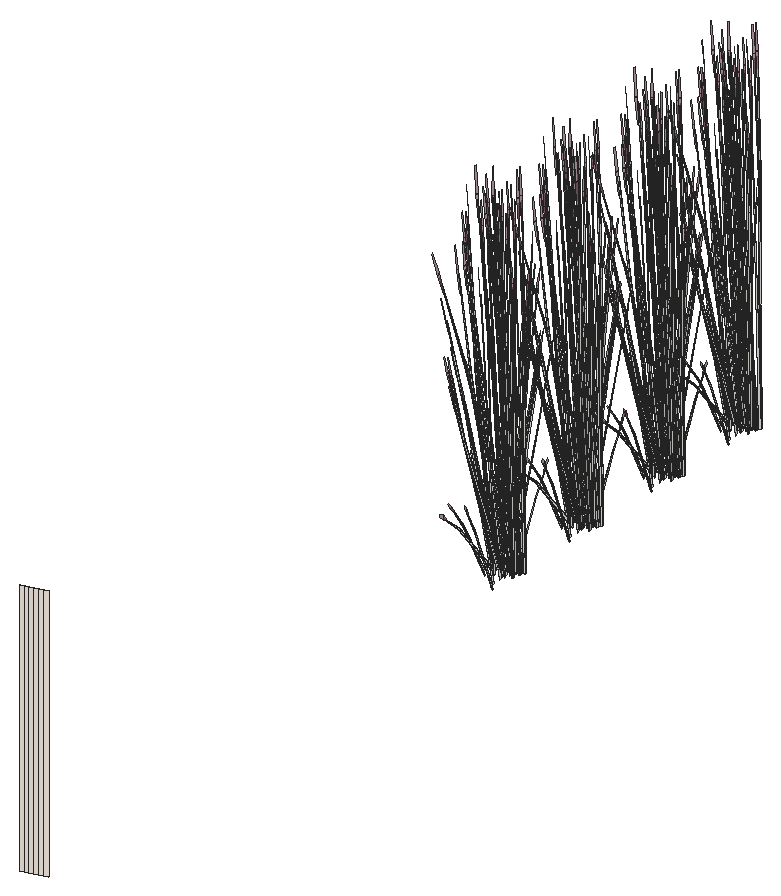
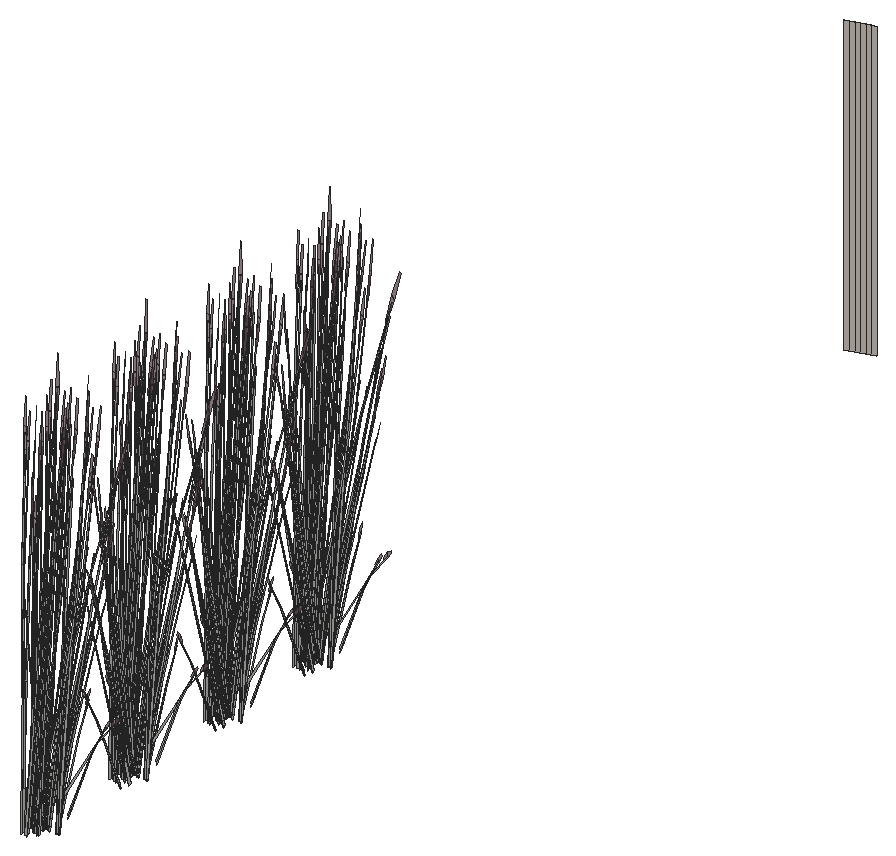
# SketchUp Ruby script. Lengths in inches.
U = 1.inch
M = Sketchup.active_model
def pt(a) = Geom::Point3d.new(a.map { |v| v * U })
def face(e, loops, mat)
  f = e.add_face(loops[0].map { |a| pt(a) })
  loops[1..].each { |l| e.add_face(l.map { |a| pt(a) }).erase! }
  f.material = f.back_material = mat if mat
  f
end
# faces: each face lists its corners as indices into pts; further lists are holes
def faces(e, pts, list, mat = nil) = list.each { |f| face(e, (f[0].is_a?(Array) ? f : [f]).map { |l| l.map { |i| pts[i] } }, mat) }
# xy, xz, yz: faces in a plane at the given z, y or x. An outline is a flat list of corners, or four numbers for a rectangle; further outlines are holes
def ring(l) = l.size == 4 ? [[l[0], l[1]], [l[2], l[1]], [l[2], l[3]], [l[0], l[3]]] : l.each_slice(2).to_a
def flat(e, list, mat, &to3) = list.each { |f| face(e, (f[0].is_a?(Array) ? f : [f]).map { |l| ring(l).map { |u, v| to3.(u, v) } }, mat) }
def xy(e, z, list, mat = nil) = flat(e, list, mat) { |x, y| [x, y, z] }
def xz(e, y, list, mat = nil) = flat(e, list, mat) { |x, z| [x, y, z] }
def yz(e, x, list, mat = nil) = flat(e, list, mat) { |y, z| [x, y, z] }
def lines(e, pts, list) = list.each { |a, b| e.add_line(pt(pts[a]), pt(pts[b])) }
# prism: a flat outline (further loops are holes) pulled along v
def prism(e, loops, v, mat = nil)
  f = face(e, loops, mat); d = Geom::Vector3d.new(v.map { |x| x * U })
  f.pushpull(f.normal.samedirection?(d) ? d.length : -d.length)
end
def box(e, o, s, mat = nil) = prism(e, [[o, [o[0] + s[0], o[1], o[2]], [o[0] + s[0], o[1] + s[1], o[2]], [o[0], o[1] + s[1], o[2]]]], [0, 0, s[2]], mat)
def at(x, y, z, deg = 0) = Geom::Transformation.translation(pt([x, y, z])) * Geom::Transformation.rotation(ORIGIN, Z_AXIS, deg.degrees)
def axes(o, x, y, z) = Geom::Transformation.new([*x, 0, *y, 0, *z, 0, *pt(o).to_a, 1])
def part(name) = M.definitions.add(name)
# library, detail: a bought-in or finely detailed component or shape, given as its bounding box
def library(name, o, s) = part(name).tap { |d| box(d.entities, o, s) }
def detail(e, o, s) = box(e.add_group.entities, o, s)
def put(e, d, t, mat = nil) = e.add_instance(d, t).tap { |i| i.material = mat if mat }
def group(e, t, mat = nil) = e.add_group.tap { |g| g.transformation = t; g.material = mat if mat }.entities
root = M.entities
M.materials.add("C01_Vanilla_Cream").color = [255, 246, 235]
M.materials.add("LightPink_Translucent").color = [144, 107, 117]
M.materials["LightPink_Translucent"].alpha = 0.75
c1 = part("blade")
p = [[2.15,0.21,22],[0,0.17,0],[0.09,0.45,0],[2.18,0.31,22],[2.29,0.31,22],[0.38,0.45,0],
  [2.48,0.24,33],[2.49,0.24,33],[2.48,0.22,33]]
faces(c1.entities,p,[[0,1,2,3],[4,5,2,3],[6,3,4,7],[8,0,3,6]])
c2 = part("seeds")
p = [[0.3,-0.1,1.38],[-0.01,-0.03,1.59],[-0.01,-0.03,0.03],[0.14,-0.07,-0.07],[0.29,-0.03,3],[0.15,0.01,3.11]]
faces(c2.entities,p,[[0,1,2,3],[1,0,4,5]],"LightPink_Translucent")
c3 = part("blade with seeds")
put(c3.entities,c1,at(0,0,0))
put(c3.entities,c2,axes([2.4,0.25,30.99],[1.5799,-0.05474,1.17369],[-0.12525,1.92788,0.29478],[-0.07173,-0.02425,1.56792]))
p = [[339.93,12.43,654],[339.37,12.32,654],[339.37,12.32,690],[339.93,12.43,690],[340.48,12.57,654],[340.48,12.57,690],
  [341.02,12.71,654],[341.02,12.71,690],[341.5625,12.88,654],[341.5625,12.88,690],[342.1,13.0625,654],[342.1,13.0625,690],
  [342.625,13.26,654],[342.625,13.26,690]]
faces(root,p,[[0,1,2,3],[4,0,3,5],[6,4,5,7],[8,6,7,9],[10,8,9,11],[12,10,11,13]],"C01_Vanilla_Cream")
put(root,c3,axes([340.5625,124.2,657.71],[-0.33433,0.21811,-0.29039],[-0.31649,-0.24905,0.3749],[-0.04815,0.12654,0.71734]))
put(root,c3,axes([342.27,95.55,655.6875],[-0.33282,0.31137,-0.51129],[-0.41344,-0.28235,-0.13419],[-0.13336,0.07767,1.12859]))
put(root,c3,axes([342.27,109.15,655.6875],[-0.33282,0.31137,-0.51129],[-0.41344,-0.28235,-0.13419],[-0.13336,0.07767,1.12859]))
put(root,c3,axes([342.27,123.55,655.6875],[-0.33282,0.31137,-0.51129],[-0.41344,-0.28235,-0.13419],[-0.13336,0.07767,1.12859]))
put(root,c3,axes([342.27,137.04,655.6875],[-0.33282,0.31137,-0.51129],[-0.41344,-0.28235,-0.13419],[-0.13336,0.07767,1.12859]))
put(root,c3,axes([341.42,93.23,658.14],[0.07631,0.33368,0.29039],[-0.43626,0.08811,-0.3749],[-0.11718,-0.09562,0.71734]))
put(root,c3,axes([341.42,106.83,658.14],[0.07631,0.33368,0.29039],[-0.43626,0.08811,-0.3749],[-0.11718,-0.09562,0.71734]))
put(root,c3,axes([341.42,121.23,658.14],[0.07631,0.33368,0.29039],[-0.43626,0.08811,-0.3749],[-0.11718,-0.09562,0.71734]))
put(root,c3,axes([341.42,134.72,658.14],[0.07631,0.33368,0.29039],[-0.43626,0.08811,-0.3749],[-0.11718,-0.09562,0.71734]))
put(root,c3,axes([339.37,96.98,657.86],[0.05606,-0.02501,1.45454],[0.46332,0.16636,-0.13744],[-0.01089,0.13852,0.2574]))
put(root,c3,axes([339.37,110.58,657.86],[0.05606,-0.02501,1.45454],[0.46332,0.16636,-0.13744],[-0.01089,0.13852,0.2574]))
put(root,c3,axes([339.37,124.97,657.86],[0.05606,-0.02501,1.45454],[0.46332,0.16636,-0.13744],[-0.01089,0.13852,0.2574]))
put(root,c3,axes([340.42,94.53,655.91],[-0.45961,0.34828,0.2522],[-0.45989,-0.34462,-0.29923],[-0.01605,-0.09891,1.35206]))
put(root,c3,axes([340.42,108.13,655.91],[-0.45961,0.34828,0.2522],[-0.45989,-0.34462,-0.29923],[-0.01605,-0.09891,1.35206]))
put(root,c3,axes([340.42,122.52,655.91],[-0.45961,0.34828,0.2522],[-0.45989,-0.34462,-0.29923],[-0.01605,-0.09891,1.35206]))
put(root,c3,axes([340.42,136.01,655.91],[-0.45961,0.34828,0.2522],[-0.45989,-0.34462,-0.29923],[-0.01605,-0.09891,1.35206]))
put(root,c3,axes([342.3125,95.49,656.73],[0.427,0.16705,1.24034],[-0.41831,0.35988,0.49049],[-0.18737,-0.21329,1.03981]))
put(root,c3,axes([342.3125,109.09,656.73],[0.427,0.16705,1.24034],[-0.41831,0.35988,0.49049],[-0.18737,-0.21329,1.03981]))
put(root,c3,axes([342.3125,123.49,656.73],[0.427,0.16705,1.24034],[-0.41831,0.35988,0.49049],[-0.18737,-0.21329,1.03981]))
put(root,c3,axes([342.3125,136.98,656.73],[0.427,0.16705,1.24034],[-0.41831,0.35988,0.49049],[-0.18737,-0.21329,1.03981]))
put(root,c3,axes([340.68,92.46,656.27],[0.25775,0.14418,0.94186],[-0.37538,0.08667,0.69201],[-0.08032,-0.11081,0.20745]))
put(root,c3,axes([340.68,106.06,656.27],[0.25775,0.14418,0.94186],[-0.37538,0.08667,0.69201],[-0.08032,-0.11081,0.20745]))
put(root,c3,axes([340.68,120.46,656.27],[0.25775,0.14418,0.94186],[-0.37538,0.08667,0.69201],[-0.08032,-0.11081,0.20745]))
put(root,c3,axes([340.68,133.95,656.27],[0.25775,0.14418,0.94186],[-0.37538,0.08667,0.69201],[-0.08032,-0.11081,0.20745]))
put(root,c3,axes([342.5,95.375,656.02],[-0.48249,-0.33343,-0.20658],[0.406,-0.37441,0.45206],[-0.12993,0.039,1.37937]))
put(root,c3,axes([342.5,108.97,656.02],[-0.48249,-0.33343,-0.20658],[0.406,-0.37441,0.45206],[-0.12993,0.039,1.37937]))
put(root,c3,axes([342.5,123.37,656.02],[-0.48249,-0.33343,-0.20658],[0.406,-0.37441,0.45206],[-0.12993,0.039,1.37937]))
put(root,c3,axes([342.5,136.86,656.02],[-0.48249,-0.33343,-0.20658],[0.406,-0.37441,0.45206],[-0.12993,0.039,1.37937]))
put(root,c3,axes([341.625,95.06,655.8125],[-0.29683,-0.34771,-0.36686],[0.44961,-0.24485,0.17656],[-0.09606,-0.04302,1.17788]))
put(root,c3,axes([341.625,108.65,655.8125],[-0.29683,-0.34771,-0.36686],[0.44961,-0.24485,0.17656],[-0.09606,-0.04302,1.17788]))
put(root,c3,axes([341.625,123.05,655.8125],[-0.29683,-0.34771,-0.36686],[0.44961,-0.24485,0.17656],[-0.09606,-0.04302,1.17788]))
put(root,c3,axes([341.625,136.54,655.8125],[-0.29683,-0.34771,-0.36686],[0.44961,-0.24485,0.17656],[-0.09606,-0.04302,1.17788]))
put(root,c3,axes([340.78,95.97,658.38],[-0.01286,0.38319,-0.64665],[-0.54141,-0.02574,0.07804],[-0.05714,0.16234,0.91476]))
put(root,c3,axes([340.78,109.57,658.38],[-0.01286,0.38319,-0.64665],[-0.54141,-0.02574,0.07804],[-0.05714,0.16234,0.91476]))
put(root,c3,axes([340.78,123.97,658.38],[-0.01286,0.38319,-0.64665],[-0.54141,-0.02574,0.07804],[-0.05714,0.16234,0.91476]))
put(root,c3,axes([340.77,97.05,656.27],[-0.01279,-0.24632,0.94186],[0.31954,0.17569,0.69201],[-0.06284,0.11741,0.20745]))
put(root,c3,axes([340.77,110.65,656.27],[-0.01279,-0.24632,0.94186],[0.31954,0.17569,0.69201],[-0.06284,0.11741,0.20745]))
put(root,c3,axes([340.77,125.05,656.27],[-0.01279,-0.24632,0.94186],[0.31954,0.17569,0.69201],[-0.06284,0.11741,0.20745]))
put(root,c3,axes([341.22,92.84,658.18],[0.55043,-0.10648,0.44086],[0.09553,0.41768,0.3635],[-0.12945,-0.1231,0.91224]))
put(root,c3,axes([341.22,106.4375,658.18],[0.55043,-0.10648,0.44086],[0.09553,0.41768,0.3635],[-0.12945,-0.1231,0.91224]))
put(root,c3,axes([341.22,120.83,658.18],[0.55043,-0.10648,0.44086],[0.09553,0.41768,0.3635],[-0.12945,-0.1231,0.91224]))
put(root,c3,axes([341.22,134.33,658.18],[0.55043,-0.10648,0.44086],[0.09553,0.41768,0.3635],[-0.12945,-0.1231,0.91224]))
put(root,c3,axes([342.26,95.31,655.8125],[-0.53657,0.02557,-0.36686],[-0.04852,-0.4245,0.17656],[-0.09606,0.04302,1.17788]))
put(root,c3,axes([342.26,108.9,655.8125],[-0.53657,0.02557,-0.36686],[-0.04852,-0.4245,0.17656],[-0.09606,0.04302,1.17788]))
put(root,c3,axes([342.26,123.3,655.8125],[-0.53657,0.02557,-0.36686],[-0.04852,-0.4245,0.17656],[-0.09606,0.04302,1.17788]))
put(root,c3,axes([342.26,136.79,655.8125],[-0.53657,0.02557,-0.36686],[-0.04852,-0.4245,0.17656],[-0.09606,0.04302,1.17788]))
put(root,c3,axes([341.35,92.93,657.88],[0.22457,-0.26316,0.05273],[0.3198,0.15321,0.41509],[-0.10339,-0.08437,0.63295]))
put(root,c3,axes([341.35,106.53,657.88],[0.22457,-0.26316,0.05273],[0.3198,0.15321,0.41509],[-0.10339,-0.08437,0.63295]))
put(root,c3,axes([341.35,120.92,657.88],[0.22457,-0.26316,0.05273],[0.3198,0.15321,0.41509],[-0.10339,-0.08437,0.63295]))
put(root,c3,axes([341.35,134.42,657.88],[0.22457,-0.26316,0.05273],[0.3198,0.15321,0.41509],[-0.10339,-0.08437,0.63295]))
put(root,c3,axes([341.23,96.02,656.03],[0.46245,0.20713,0.40713],[-0.27641,0.37142,0],[-0.10533,-0.04718,1.29153]))
put(root,c3,axes([341.23,109.61,656.03],[0.46245,0.20713,0.40713],[-0.27641,0.37142,0],[-0.10533,-0.04718,1.29153]))
put(root,c3,axes([341.23,124.01,656.03],[0.46245,0.20713,0.40713],[-0.27641,0.37142,0],[-0.10533,-0.04718,1.29153]))
put(root,c3,axes([341.23,137.5,656.03],[0.46245,0.20713,0.40713],[-0.27641,0.37142,0],[-0.10533,-0.04718,1.29153]))
put(root,c3,axes([340.6,96.51,656.76],[0.01086,-0.21386,1.26563],[0.48828,0.11296,0.1749],[-0.04231,0.22792,0.59763]))
put(root,c3,axes([340.6,110.11,656.76],[0.01086,-0.21386,1.26563],[0.48828,0.11296,0.1749],[-0.04231,0.22792,0.59763]))
put(root,c3,axes([340.6,124.51,656.76],[0.01086,-0.21386,1.26563],[0.48828,0.11296,0.1749],[-0.04231,0.22792,0.59763]))
put(root,c3,axes([341.67,95.26,656],[0.13096,-0.49088,-0.19212],[0.62096,0.08557,0.42042],[-0.1085,-0.06779,1.28281]))
put(root,c3,axes([341.67,108.85,656],[0.13096,-0.49088,-0.19212],[0.62096,0.08557,0.42042],[-0.1085,-0.06779,1.28281]))
put(root,c3,axes([341.67,123.25,656],[0.13096,-0.49088,-0.19212],[0.62096,0.08557,0.42042],[-0.1085,-0.06779,1.28281]))
put(root,c3,axes([341.67,136.74,656],[0.13096,-0.49088,-0.19212],[0.62096,0.08557,0.42042],[-0.1085,-0.06779,1.28281]))
put(root,c3,axes([341.89,95.37,656.15],[-0.09532,0.36971,0.11873],[-0.46572,-0.06418,-0.33905],[-0.08476,-0.03796,1.0393]))
put(root,c3,axes([341.89,108.97,656.15],[-0.09532,0.36971,0.11873],[-0.46572,-0.06418,-0.33905],[-0.08476,-0.03796,1.0393]))
put(root,c3,axes([341.89,123.36,656.15],[-0.09532,0.36971,0.11873],[-0.46572,-0.06418,-0.33905],[-0.08476,-0.03796,1.0393]))
put(root,c3,axes([341.89,136.86,656.15],[-0.09532,0.36971,0.11873],[-0.46572,-0.06418,-0.33905],[-0.08476,-0.03796,1.0393]))
put(root,c3,axes([341.84,92.15,657.87],[-0.07558,-0.05808,1.43454],[-0.50436,0.03682,-0.22687],[-0.08049,-0.13892,0.11505]))
put(root,c3,axes([341.84,105.75,657.87],[-0.07558,-0.05808,1.43454],[-0.50436,0.03682,-0.22687],[-0.08049,-0.13892,0.11505]))
put(root,c3,axes([341.84,120.14,657.87],[-0.07558,-0.05808,1.43454],[-0.50436,0.03682,-0.22687],[-0.08049,-0.13892,0.11505]))
put(root,c3,axes([341.84,133.63,657.87],[-0.07558,-0.05808,1.43454],[-0.50436,0.03682,-0.22687],[-0.08049,-0.13892,0.11505]))
put(root,c3,axes([342.82,96.4,655.65],[-0.46245,0.20713,-0.40713],[-0.27641,-0.37142,0],[-0.10533,0.04718,1.29153]))
put(root,c3,axes([342.82,110,655.65],[-0.46245,0.20713,-0.40713],[-0.27641,-0.37142,0],[-0.10533,0.04718,1.29153]))
put(root,c3,axes([342.82,124.39,655.65],[-0.46245,0.20713,-0.40713],[-0.27641,-0.37142,0],[-0.10533,0.04718,1.29153]))
put(root,c3,axes([342.82,137.89,655.65],[-0.46245,0.20713,-0.40713],[-0.27641,-0.37142,0],[-0.10533,0.04718,1.29153]))
put(root,c3,axes([340.08,94.34,655.65],[0,-0.41426,-0.40713],[0.55282,0,0],[0,-0.09435,1.29153]))
put(root,c3,axes([340.08,107.94,655.65],[0,-0.41426,-0.40713],[0.55282,0,0],[0,-0.09435,1.29153]))
put(root,c3,axes([340.08,122.33,655.65],[0,-0.41426,-0.40713],[0.55282,0,0],[0,-0.09435,1.29153]))
put(root,c3,axes([340.08,135.82,655.65],[0,-0.41426,-0.40713],[0.55282,0,0],[0,-0.09435,1.29153]))
put(root,c3,axes([340.32,94.72,656.03],[0,0.41426,0.40713],[-0.55282,0,0],[0,-0.09435,1.29153]))
put(root,c3,axes([340.32,108.32,656.03],[0,0.41426,0.40713],[-0.55282,0,0],[0,-0.09435,1.29153]))
put(root,c3,axes([340.32,122.72,656.03],[0,0.41426,0.40713],[-0.55282,0,0],[0,-0.09435,1.29153]))
put(root,c3,axes([340.32,136.21,656.03],[0,0.41426,0.40713],[-0.55282,0,0],[0,-0.09435,1.29153]))
put(root,c3,axes([342.85,96.29,655.8],[-0.30508,-0.41657,-0.04217],[0.51685,-0.2315,0.42318],[-0.12736,0.03966,1.34177]))
put(root,c3,axes([342.85,109.89,655.8],[-0.30508,-0.41657,-0.04217],[0.51685,-0.2315,0.42318],[-0.12736,0.03966,1.34177]))
put(root,c3,axes([342.85,124.28,655.8],[-0.30508,-0.41657,-0.04217],[0.51685,-0.2315,0.42318],[-0.12736,0.03966,1.34177]))
put(root,c3,axes([342.85,137.77,655.8],[-0.30508,-0.41657,-0.04217],[0.51685,-0.2315,0.42318],[-0.12736,0.03966,1.34177]))
put(root,c3,axes([340.89,96.1,658.1],[0.35372,0.27835,-0.4651],[-0.37366,0.24377,-0.36026],[-0.05382,0.14142,0.88993]))
put(root,c3,axes([340.89,109.7,658.1],[0.35372,0.27835,-0.4651],[-0.37366,0.24377,-0.36026],[-0.05382,0.14142,0.88993]))
put(root,c3,axes([340.89,124.1,658.1],[0.35372,0.27835,-0.4651],[-0.37366,0.24377,-0.36026],[-0.05382,0.14142,0.88993]))
put(root,c3,axes([342.71,96.24,655.66],[-0.46099,-0.1025,-0.25402],[0.11607,-0.36097,0.25402],[-0.09293,0.04163,1.13959]))
put(root,c3,axes([342.71,109.84,655.66],[-0.46099,-0.1025,-0.25402],[0.11607,-0.36097,0.25402],[-0.09293,0.04163,1.13959]))
put(root,c3,axes([342.71,124.23,655.66],[-0.46099,-0.1025,-0.25402],[0.11607,-0.36097,0.25402],[-0.09293,0.04163,1.13959]))
put(root,c3,axes([342.71,137.72,655.66],[-0.46099,-0.1025,-0.25402],[0.11607,-0.36097,0.25402],[-0.09293,0.04163,1.13959]))
put(root,c3,axes([340.74,95.89,658.14],[0.33433,-0.21811,0.29039],[0.31649,0.24905,-0.3749],[-0.04815,0.12654,0.71734]))
put(root,c3,axes([340.74,109.49,658.14],[0.33433,-0.21811,0.29039],[0.31649,0.24905,-0.3749],[-0.04815,0.12654,0.71734]))
put(root,c3,axes([340.74,123.89,658.14],[0.33433,-0.21811,0.29039],[0.31649,0.24905,-0.3749],[-0.04815,0.12654,0.71734]))
put(root,c3,axes([340.74,137.38,658.14],[0.33433,-0.21811,0.29039],[0.31649,0.24905,-0.3749],[-0.04815,0.12654,0.71734]))
put(root,c3,axes([341.53,94.82,656.1875],[-0.55647,-0.19766,-0.23858],[0.26794,-0.4172,-0.41002],[-0.01749,-0.10243,1.3096]))
put(root,c3,axes([341.53,108.41,656.1875],[-0.55647,-0.19766,-0.23858],[0.26794,-0.4172,-0.41002],[-0.01749,-0.10243,1.3096]))
put(root,c3,axes([341.53,122.81,656.1875],[-0.55647,-0.19766,-0.23858],[0.26794,-0.4172,-0.41002],[-0.01749,-0.10243,1.3096]))
put(root,c3,axes([341.53,136.3,656.1875],[-0.55647,-0.19766,-0.23858],[0.26794,-0.4172,-0.41002],[-0.01749,-0.10243,1.3096]))
put(root,c3,axes([342.98,94.69,656.33],[-0.0135,-0.39004,1.15843],[0.61089,0.10111,0.49049],[-0.14449,0.21343,1.09347]))
put(root,c3,axes([342.98,108.29,656.33],[-0.0135,-0.39004,1.15843],[0.61089,0.10111,0.49049],[-0.14449,0.21343,1.09347]))
put(root,c3,axes([342.98,122.6875,656.33],[-0.0135,-0.39004,1.15843],[0.61089,0.10111,0.49049],[-0.14449,0.21343,1.09347]))
put(root,c3,axes([342.98,136.18,656.33],[-0.0135,-0.39004,1.15843],[0.61089,0.10111,0.49049],[-0.14449,0.21343,1.09347]))
put(root,c3,axes([340.52,95.95,658.43],[0.54305,0.02053,-0.11068],[-0.01484,0.38862,-0.61434],[-0.03772,0.14967,0.93347]))
put(root,c3,axes([340.52,109.55,658.43],[0.54305,0.02053,-0.11068],[-0.01484,0.38862,-0.61434],[-0.03772,0.14967,0.93347]))
put(root,c3,axes([340.52,123.95,658.43],[0.54305,0.02053,-0.11068],[-0.01484,0.38862,-0.61434],[-0.03772,0.14967,0.93347]))
put(root,c3,axes([340.51,96.52,656.31],[0.44888,-0.07336,0.05336],[0.1032,0.29555,-0.7077],[-0.02846,0.14961,0.63435]))
put(root,c3,axes([340.51,110.12,656.31],[0.44888,-0.07336,0.05336],[0.1032,0.29555,-0.7077],[-0.02846,0.14961,0.63435]))
put(root,c3,axes([340.51,124.51,656.31],[0.44888,-0.07336,0.05336],[0.1032,0.29555,-0.7077],[-0.02846,0.14961,0.63435]))
put(root,c3,axes([342.63,95.19,656.1875],[0.05758,0.4727,-0.23858],[-0.59969,0.02858,-0.41002],[-0.1056,0.06296,1.3096]))
put(root,c3,axes([342.63,108.79,656.1875],[0.05758,0.4727,-0.23858],[-0.59969,0.02858,-0.41002],[-0.1056,0.06296,1.3096]))
put(root,c3,axes([342.63,123.18,656.1875],[0.05758,0.4727,-0.23858],[-0.59969,0.02858,-0.41002],[-0.1056,0.06296,1.3096]))
put(root,c3,axes([342.63,136.67,656.1875],[0.05758,0.4727,-0.23858],[-0.59969,0.02858,-0.41002],[-0.1056,0.06296,1.3096]))
put(root,c3,axes([341.28,94.4,655.72],[-0.20292,-0.42481,-0.57265],[0.58453,-0.15299,-0.1503],[-0.02243,-0.14385,1.26402]))
put(root,c3,axes([341.28,107.99,655.72],[-0.20292,-0.42481,-0.57265],[0.58453,-0.15299,-0.1503],[-0.02243,-0.14385,1.26402]))
put(root,c3,axes([341.28,122.39,655.72],[-0.20292,-0.42481,-0.57265],[0.58453,-0.15299,-0.1503],[-0.02243,-0.14385,1.26402]))
put(root,c3,axes([341.28,135.88,655.72],[-0.20292,-0.42481,-0.57265],[0.58453,-0.15299,-0.1503],[-0.02243,-0.14385,1.26402]))
put(root,c3,axes([342.61,93.05,658.13],[-0.48353,0.19287,-0.09971],[-0.23761,-0.34232,-0.55346],[-0.0638,-0.14425,0.84097]))
put(root,c3,axes([342.61,106.64,658.13],[-0.48353,0.19287,-0.09971],[-0.23761,-0.34232,-0.55346],[-0.0638,-0.14425,0.84097]))
put(root,c3,axes([342.61,121.04,658.13],[-0.48353,0.19287,-0.09971],[-0.23761,-0.34232,-0.55346],[-0.0638,-0.14425,0.84097]))
put(root,c3,axes([342.61,134.53,658.13],[-0.48353,0.19287,-0.09971],[-0.23761,-0.34232,-0.55346],[-0.0638,-0.14425,0.84097]))
put(root,c3,axes([342.19,93.0625,657.84],[-0.48573,-0.10385,-0.41901],[0.16649,-0.35605,-0.32456],[-0.04454,-0.14335,0.80174]))
put(root,c3,axes([342.19,106.66,657.84],[-0.48573,-0.10385,-0.41901],[0.16649,-0.35605,-0.32456],[-0.04454,-0.14335,0.80174]))
put(root,c3,axes([342.19,121.06,657.84],[-0.48573,-0.10385,-0.41901],[0.16649,-0.35605,-0.32456],[-0.04454,-0.14335,0.80174]))
put(root,c3,axes([342.19,134.55,657.84],[-0.48573,-0.10385,-0.41901],[0.16649,-0.35605,-0.32456],[-0.04454,-0.14335,0.80174]))
put(root,c3,axes([341.3,95.7,657.18],[-0.01209,-0.159,1.40529],[0.52417,0.10548,0.11363],[-0.03242,0.22659,0.60075]))
put(root,c3,axes([341.3,109.3,657.18],[-0.01209,-0.159,1.40529],[0.52417,0.10548,0.11363],[-0.03242,0.22659,0.60075]))
put(root,c3,axes([341.3,123.7,657.18],[-0.01209,-0.159,1.40529],[0.52417,0.10548,0.11363],[-0.03242,0.22659,0.60075]))
put(root,c3,axes([340.32,94.35,655.66],[0.34492,-0.25847,-0.25402],[0.34492,0.25847,0.25402],[0,-0.08325,1.13959]))
put(root,c3,axes([340.32,107.94,655.66],[0.34492,-0.25847,-0.25402],[0.34492,0.25847,0.25402],[0,-0.08325,1.13959]))
put(root,c3,axes([340.32,122.34,655.66],[0.34492,-0.25847,-0.25402],[0.34492,0.25847,0.25402],[0,-0.08325,1.13959]))
put(root,c3,axes([340.32,135.83,655.66],[0.34492,-0.25847,-0.25402],[0.34492,0.25847,0.25402],[0,-0.08325,1.13959]))
put(root,c3,axes([341.875,92.67,655.74],[-0.34145,0.23766,-0.03192],[-0.31287,-0.26029,-0.14473],[-0.02203,-0.07375,0.47736]))
put(root,c3,axes([341.875,106.27,655.74],[-0.34145,0.23766,-0.03192],[-0.31287,-0.26029,-0.14473],[-0.02203,-0.07375,0.47736]))
put(root,c3,axes([341.875,120.67,655.74],[-0.34145,0.23766,-0.03192],[-0.31287,-0.26029,-0.14473],[-0.02203,-0.07375,0.47736]))
put(root,c3,axes([341.875,134.16,655.74],[-0.34145,0.23766,-0.03192],[-0.31287,-0.26029,-0.14473],[-0.02203,-0.07375,0.47736]))
put(root,c3,axes([341.74,95.02,655.9375],[0.62452,0.08728,0.37519],[-0.1271,0.49295,0.14723],[-0.09127,-0.0476,1.30262]))
put(root,c3,axes([341.74,108.62,655.9375],[0.62452,0.08728,0.37519],[-0.1271,0.49295,0.14723],[-0.09127,-0.0476,1.30262]))
put(root,c3,axes([341.74,123.01,655.9375],[0.62452,0.08728,0.37519],[-0.1271,0.49295,0.14723],[-0.09127,-0.0476,1.30262]))
put(root,c3,axes([341.74,136.5,655.9375],[0.62452,0.08728,0.37519],[-0.1271,0.49295,0.14723],[-0.09127,-0.0476,1.30262]))
put(root,c3,axes([341.58,94.93,656.23],[-0.23974,0.37328,0.36686],[-0.49814,-0.17965,-0.17656],[0,-0.08605,1.17788]))
put(root,c3,axes([341.58,108.53,656.23],[-0.23974,0.37328,0.36686],[-0.49814,-0.17965,-0.17656],[0,-0.08605,1.17788]))
put(root,c3,axes([341.58,122.92,656.23],[-0.23974,0.37328,0.36686],[-0.49814,-0.17965,-0.17656],[0,-0.08605,1.17788]))
put(root,c3,axes([341.58,136.41,656.23],[-0.23974,0.37328,0.36686],[-0.49814,-0.17965,-0.17656],[0,-0.08605,1.17788]))
put(root,c3,axes([342.37,93.13,658.08],[-0.23583,-0.33684,-0.58257],[0.48546,-0.18772,0.0703],[-0.05515,-0.16275,0.8241]))
put(root,c3,axes([342.37,106.73,658.08],[-0.23583,-0.33684,-0.58257],[0.48546,-0.18772,0.0703],[-0.05515,-0.16275,0.8241]))
put(root,c3,axes([342.37,121.125,658.08],[-0.23583,-0.33684,-0.58257],[0.48546,-0.18772,0.0703],[-0.05515,-0.16275,0.8241]))
put(root,c3,axes([342.37,134.62,658.08],[-0.23583,-0.33684,-0.58257],[0.48546,-0.18772,0.0703],[-0.05515,-0.16275,0.8241]))
put(root,c3,axes([341.4,95.81,656.03],[0.53096,-0.10995,0.14467],[0.13111,0.40919,0.28771],[-0.04735,-0.05962,1.31534]))
put(root,c3,axes([341.4,109.4,656.03],[0.53096,-0.10995,0.14467],[0.13111,0.40919,0.28771],[-0.04735,-0.05962,1.31534]))
put(root,c3,axes([341.4,123.8,656.03],[0.53096,-0.10995,0.14467],[0.13111,0.40919,0.28771],[-0.04735,-0.05962,1.31534]))
put(root,c3,axes([341.4,137.29,656.03],[0.53096,-0.10995,0.14467],[0.13111,0.40919,0.28771],[-0.04735,-0.05962,1.31534]))
put(root,c3,axes([342.09,95.87,655.8],[-0.49814,-0.18599,0],[0.23974,-0.38645,0],[0,0,1.3342]))
put(root,c3,axes([342.09,109.47,655.8],[-0.49814,-0.18599,0],[0.23974,-0.38645,0],[0,0,1.3342]))
put(root,c3,axes([342.09,123.87,655.8],[-0.49814,-0.18599,0],[0.23974,-0.38645,0],[0,0,1.3342]))
put(root,c3,axes([342.09,137.36,655.8],[-0.49814,-0.18599,0],[0.23974,-0.38645,0],[0,0,1.3342]))
put(root,c3,axes([342.46,93.18,658.14],[-0.14896,0.31857,0.29039],[-0.4346,-0.09292,-0.3749],[-0.03985,-0.12826,0.71734]))
put(root,c3,axes([342.46,106.78,658.14],[-0.14896,0.31857,0.29039],[-0.4346,-0.09292,-0.3749],[-0.03985,-0.12826,0.71734]))
put(root,c3,axes([342.46,121.17,658.14],[-0.14896,0.31857,0.29039],[-0.4346,-0.09292,-0.3749],[-0.03985,-0.12826,0.71734]))
put(root,c3,axes([342.46,134.66,658.14],[-0.14896,0.31857,0.29039],[-0.4346,-0.09292,-0.3749],[-0.03985,-0.12826,0.71734]))
put(root,c3,axes([343.24,96.34,655.95],[0.30893,0.41511,0],[-0.51685,0.2315,-0.42318],[-0.11772,0.05273,1.34243]))
put(root,c3,axes([343.24,109.93,655.95],[0.30893,0.41511,0],[-0.51685,0.2315,-0.42318],[-0.11772,0.05273,1.34243]))
put(root,c3,axes([343.24,124.33,655.95],[0.30893,0.41511,0],[-0.51685,0.2315,-0.42318],[-0.11772,0.05273,1.34243]))
put(root,c3,axes([343.24,137.82,655.95],[0.30893,0.41511,0],[-0.51685,0.2315,-0.42318],[-0.11772,0.05273,1.34243]))
put(root,c3,axes([341.67,96.52,658.15],[-0.48688,-0.1083,0.43692],[0.16649,-0.35605,0.36026],[0.02926,0.14002,0.9041]))
put(root,c3,axes([341.67,110.11,658.15],[-0.48688,-0.1083,0.43692],[0.16649,-0.35605,0.36026],[0.02926,0.14002,0.9041]))
put(root,c3,axes([341.67,124.51,658.15],[-0.48688,-0.1083,0.43692],[0.16649,-0.35605,0.36026],[0.02926,0.14002,0.9041]))
put(root,c3,axes([341.54,96.54,657.88],[-0.36409,0.14079,0.05273],[-0.17821,-0.25674,0.41509],[0.03516,0.11317,0.63295]))
put(root,c3,axes([341.54,110.14,657.88],[-0.36409,0.14079,0.05273],[-0.17821,-0.25674,0.41509],[0.03516,0.11317,0.63295]))
put(root,c3,axes([341.54,124.54,657.88],[-0.36409,0.14079,0.05273],[-0.17821,-0.25674,0.41509],[0.03516,0.11317,0.63295]))
put(root,c3,axes([342.98,95.83,656.03],[0.14274,-0.41171,0.14467],[0.52234,0.11651,0.28771],[-0.09023,0.00201,1.31534]))
put(root,c3,axes([342.98,109.43,656.03],[0.14274,-0.41171,0.14467],[0.52234,0.11651,0.28771],[-0.09023,0.00201,1.31534]))
put(root,c3,axes([342.98,123.82,656.03],[0.14274,-0.41171,0.14467],[0.52234,0.11651,0.28771],[-0.09023,0.00201,1.31534]))
put(root,c3,axes([342.98,137.3125,656.03],[0.14274,-0.41171,0.14467],[0.52234,0.11651,0.28771],[-0.09023,0.00201,1.31534]))
put(root,c3,axes([342.74,95.28,656.15],[0.36505,0.2489,0.11873],[-0.3045,0.28081,-0.33905],[-0.08476,0.03796,1.0393]))
put(root,c3,axes([342.74,108.88,656.15],[0.36505,0.2489,0.11873],[-0.3045,0.28081,-0.33905],[-0.08476,0.03796,1.0393]))
put(root,c3,axes([342.74,123.28,656.15],[0.36505,0.2489,0.11873],[-0.3045,0.28081,-0.33905],[-0.08476,0.03796,1.0393]))
put(root,c3,axes([342.74,136.77,656.15],[0.36505,0.2489,0.11873],[-0.3045,0.28081,-0.33905],[-0.08476,0.03796,1.0393]))
put(root,c3,axes([342.61,94.98,655.88],[-0.45961,-0.35656,-0.05027],[0.45989,-0.35678,0],[-0.01605,-0.01245,1.43968]))
put(root,c3,axes([342.61,108.57,655.88],[-0.45961,-0.35656,-0.05027],[0.45989,-0.35678,0],[-0.01605,-0.01245,1.43968]))
put(root,c3,axes([342.61,122.97,655.88],[-0.45961,-0.35656,-0.05027],[0.45989,-0.35678,0],[-0.01605,-0.01245,1.43968]))
put(root,c3,axes([342.61,136.46,655.88],[-0.45961,-0.35656,-0.05027],[0.45989,-0.35678,0],[-0.01605,-0.01245,1.43968]))
put(root,c3,axes([342.73,95.1,656.23],[0.53657,-0.02557,0.36686],[0.04852,0.4245,-0.17656],[-0.09606,0.04302,1.17788]))
put(root,c3,axes([342.73,108.7,656.23],[0.53657,-0.02557,0.36686],[0.04852,0.4245,-0.17656],[-0.09606,0.04302,1.17788]))
put(root,c3,axes([342.73,123.09,656.23],[0.53657,-0.02557,0.36686],[0.04852,0.4245,-0.17656],[-0.09606,0.04302,1.17788]))
put(root,c3,axes([342.73,136.58,656.23],[0.53657,-0.02557,0.36686],[0.04852,0.4245,-0.17656],[-0.09606,0.04302,1.17788]))
put(root,c3,axes([342.86,96.08,655.91],[0.6186,0.13465,0.2522],[-0.15476,0.48129,-0.29923],[-0.10239,0.06024,1.35206]))
put(root,c3,axes([342.86,109.67,655.91],[0.6186,0.13465,0.2522],[-0.15476,0.48129,-0.29923],[-0.10239,0.06024,1.35206]))
put(root,c3,axes([342.86,124.07,655.91],[0.6186,0.13465,0.2522],[-0.15476,0.48129,-0.29923],[-0.10239,0.06024,1.35206]))
put(root,c3,axes([342.86,137.56,655.91],[0.6186,0.13465,0.2522],[-0.15476,0.48129,-0.29923],[-0.10239,0.06024,1.35206]))
put(root,c3,axes([341.96,92.38,655.22],[-0.08288,0.01493,1.44601],[-0.45833,-0.16801,-0.2209],[0.00769,-0.14014,0.2463]))
put(root,c3,axes([341.96,105.98,655.22],[-0.08288,0.01493,1.44601],[-0.45833,-0.16801,-0.2209],[0.00769,-0.14014,0.2463]))
put(root,c3,axes([341.96,120.38,655.22],[-0.08288,0.01493,1.44601],[-0.45833,-0.16801,-0.2209],[0.00769,-0.14014,0.2463]))
put(root,c3,axes([341.96,133.87,655.22],[-0.08288,0.01493,1.44601],[-0.45833,-0.16801,-0.2209],[0.00769,-0.14014,0.2463]))
put(root,c3,axes([343.13,96.05,656.03],[0.46245,-0.20713,0.40713],[0.27641,0.37142,0],[-0.10533,0.04718,1.29153]))
put(root,c3,axes([343.13,109.65,656.03],[0.46245,-0.20713,0.40713],[0.27641,0.37142,0],[-0.10533,0.04718,1.29153]))
put(root,c3,axes([343.13,124.04,656.03],[0.46245,-0.20713,0.40713],[0.27641,0.37142,0],[-0.10533,0.04718,1.29153]))
put(root,c3,axes([343.13,137.53,656.03],[0.46245,-0.20713,0.40713],[0.27641,0.37142,0],[-0.10533,0.04718,1.29153]))
put(root,c3,axes([342.41,92.84,657.71],[0.14896,-0.31857,-0.29039],[0.4346,0.09292,0.3749],[-0.03985,-0.12826,0.71734]))
put(root,c3,axes([342.41,106.44,657.71],[0.14896,-0.31857,-0.29039],[0.4346,0.09292,0.3749],[-0.03985,-0.12826,0.71734]))
put(root,c3,axes([342.41,120.84,657.71],[0.14896,-0.31857,-0.29039],[0.4346,0.09292,0.3749],[-0.03985,-0.12826,0.71734]))
put(root,c3,axes([342.41,134.33,657.71],[0.14896,-0.31857,-0.29039],[0.4346,0.09292,0.3749],[-0.03985,-0.12826,0.71734]))
put(root,c3,axes([341.69,94.56,655.9375],[0.21483,0.46323,0.37519],[-0.61383,0.16108,0.14723],[0.0075,-0.08512,1.30262]))
put(root,c3,axes([341.69,108.16,655.9375],[0.21483,0.46323,0.37519],[-0.61383,0.16108,0.14723],[0.0075,-0.08512,1.30262]))
put(root,c3,axes([341.69,122.56,655.9375],[0.21483,0.46323,0.37519],[-0.61383,0.16108,0.14723],[0.0075,-0.08512,1.30262]))
put(root,c3,axes([341.69,136.05,655.9375],[0.21483,0.46323,0.37519],[-0.61383,0.16108,0.14723],[0.0075,-0.08512,1.30262]))
put(root,c3,axes([341.59,94.51,655.8125],[0.23974,-0.37328,-0.36686],[0.49814,0.17965,0.17656],[0,-0.08605,1.17788]))
put(root,c3,axes([341.59,108.1,655.8125],[0.23974,-0.37328,-0.36686],[0.49814,0.17965,0.17656],[0,-0.08605,1.17788]))
put(root,c3,axes([341.59,122.5,655.8125],[0.23974,-0.37328,-0.36686],[0.49814,0.17965,0.17656],[0,-0.08605,1.17788]))
put(root,c3,axes([341.59,135.99,655.8125],[0.23974,-0.37328,-0.36686],[0.49814,0.17965,0.17656],[0,-0.08605,1.17788]))
put(root,c3,axes([342.2,95.71,655.81],[-0.16122,-0.35715,0],[0.46037,-0.12507,0],[0,0,1.26584]))
put(root,c3,axes([342.2,109.31,655.81],[-0.16122,-0.35715,0],[0.46037,-0.12507,0],[0,0,1.26584]))
put(root,c3,axes([342.2,123.7,655.81],[-0.16122,-0.35715,0],[0.46037,-0.12507,0],[0,0,1.26584]))
put(root,c3,axes([342.2,137.19,655.81],[-0.16122,-0.35715,0],[0.46037,-0.12507,0],[0,0,1.26584]))
put(root,c3,axes([341.61,96.46,655.22],[0.07997,-0.02254,1.44601],[0.48102,0.12407,-0.2209],[0.01407,0.13984,0.2463]))
put(root,c3,axes([341.61,110.0625,655.22],[0.07997,-0.02254,1.44601],[0.48102,0.12407,-0.2209],[0.01407,0.13984,0.2463]))
put(root,c3,axes([341.61,124.46,655.22],[0.07997,-0.02254,1.44601],[0.48102,0.12407,-0.2209],[0.01407,0.13984,0.2463]))
put(root,c3,axes([341.72,96.59,657.71],[-0.14896,0.31857,-0.29039],[-0.4346,-0.09292,0.3749],[0.03985,0.12826,0.71734]))
put(root,c3,axes([341.72,110.1875,657.71],[-0.14896,0.31857,-0.29039],[-0.4346,-0.09292,0.3749],[0.03985,0.12826,0.71734]))
put(root,c3,axes([341.72,124.58,657.71],[-0.14896,0.31857,-0.29039],[-0.4346,-0.09292,0.3749],[0.03985,0.12826,0.71734]))
put(root,c3,axes([342.85,95.01,655.8125],[-0.23974,0.37328,-0.36686],[-0.49814,-0.17965,0.17656],[0,0.08605,1.17788]))
